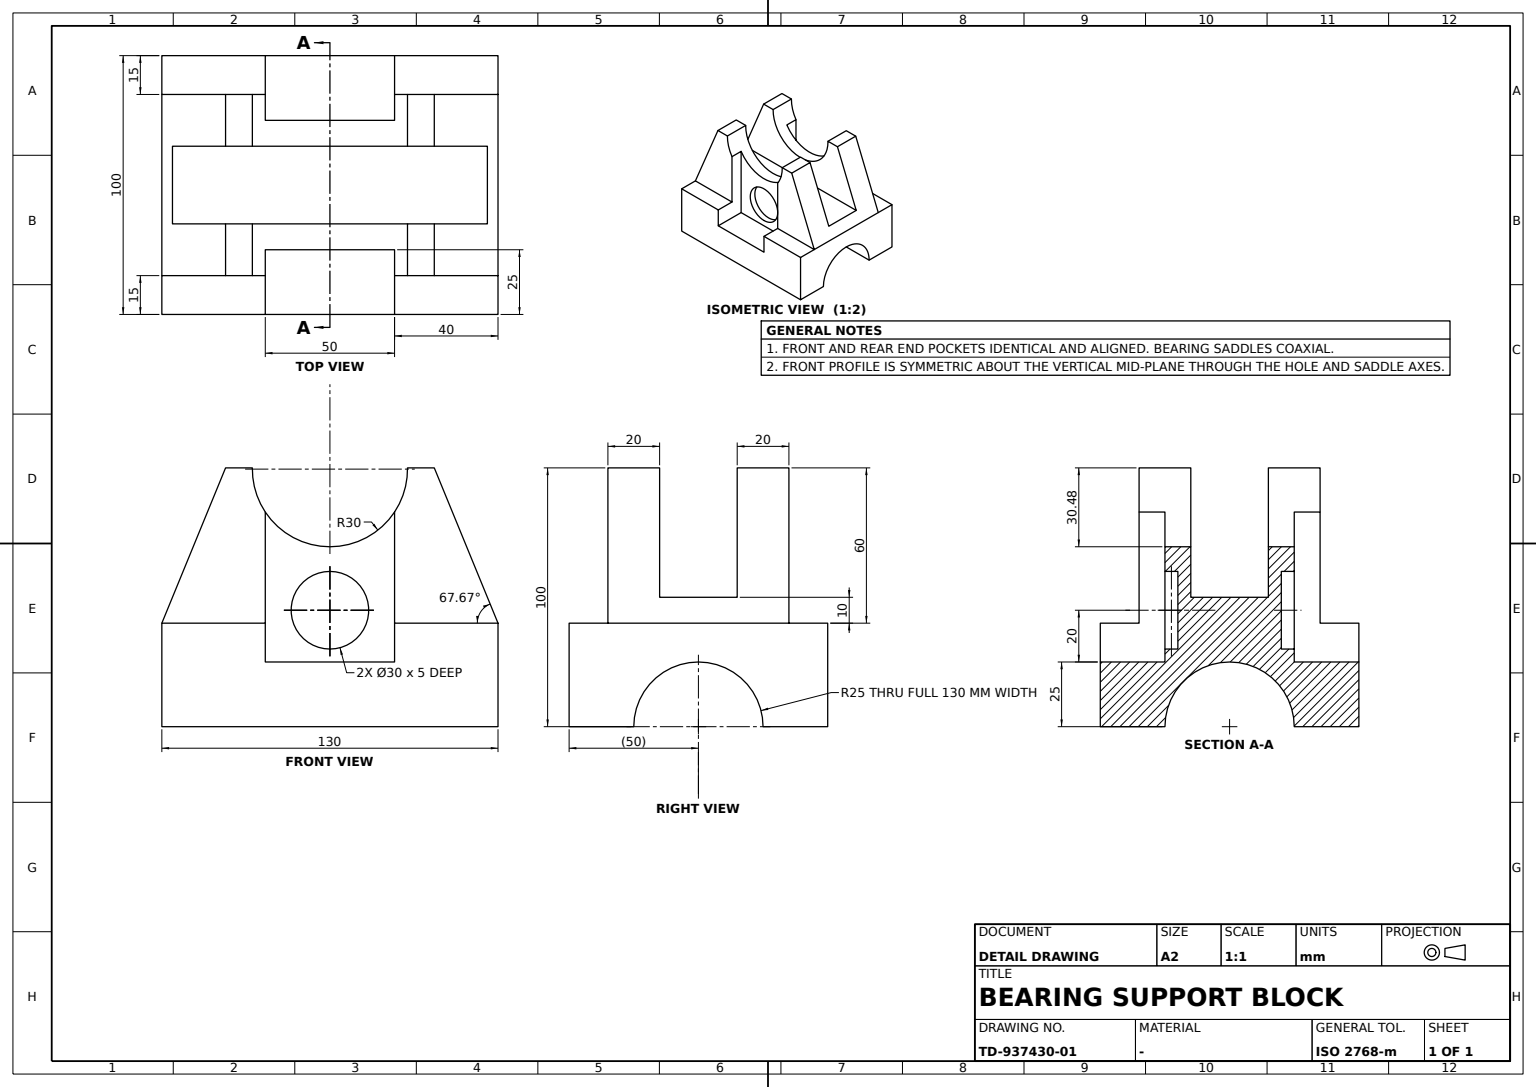
ISO-10303-21;
HEADER;
FILE_DESCRIPTION((''),'2;1');
FILE_NAME('','',(''),(''),'','','');
FILE_SCHEMA(('AUTOMOTIVE_DESIGN'));
ENDSEC;
DATA;
#1=APPLICATION_CONTEXT('');
#2=PRODUCT_CONTEXT('',#1,'mechanical');
#3=PRODUCT('','','',(#2));
#4=PRODUCT_DEFINITION_FORMATION('','',#3);
#5=PRODUCT_DEFINITION_CONTEXT('',#1,'design');
#6=PRODUCT_DEFINITION('','',#4,#5);
#7=PRODUCT_DEFINITION_SHAPE('','',#6);
#8=(LENGTH_UNIT()NAMED_UNIT(*)SI_UNIT(.MILLI.,.METRE.));
#9=(NAMED_UNIT(*)PLANE_ANGLE_UNIT()SI_UNIT($,.RADIAN.));
#10=(NAMED_UNIT(*)SI_UNIT($,.STERADIAN.)SOLID_ANGLE_UNIT());
#11=UNCERTAINTY_MEASURE_WITH_UNIT(LENGTH_MEASURE(0.005),#8,'distance_accuracy_value','');
#12=(GEOMETRIC_REPRESENTATION_CONTEXT(3)GLOBAL_UNCERTAINTY_ASSIGNED_CONTEXT((#11))GLOBAL_UNIT_ASSIGNED_CONTEXT((#8,#9,#10))REPRESENTATION_CONTEXT('',''));
#13=CARTESIAN_POINT('',(-15.,29.996182,100.));
#14=VERTEX_POINT('',#13);
#15=CARTESIAN_POINT('',(-15.,-29.996182,100.));
#16=VERTEX_POINT('',#15);
#17=CARTESIAN_POINT('',(-15.,0.,99.521385));
#18=DIRECTION('',(-1.,0.,0.));
#19=DIRECTION('',(0.,0.,1.));
#20=AXIS2_PLACEMENT_3D('',#17,#18,#19);
#21=CIRCLE('',#20,30.);
#22=EDGE_CURVE('',#14,#16,#21,.T.);
#23=ORIENTED_EDGE('',*,*,#22,.F.);
#24=CARTESIAN_POINT('',(-35.,29.996182,100.));
#25=VERTEX_POINT('',#24);
#26=DIRECTION('',(1.,0.,0.));
#27=VECTOR('',#26,1000.);
#28=LINE('',#13,#27);
#29=EDGE_CURVE('',#14,#25,#28,.F.);
#30=ORIENTED_EDGE('',*,*,#29,.T.);
#31=CARTESIAN_POINT('',(-35.,25.,82.938261));
#32=VERTEX_POINT('',#31);
#33=CARTESIAN_POINT('',(-35.,0.,99.521385));
#34=DIRECTION('',(0.,0.,-1.));
#35=AXIS2_PLACEMENT_3D('',#33,#26,#34);
#36=CIRCLE('',#35,30.);
#37=EDGE_CURVE('',#32,#25,#36,.T.);
#38=ORIENTED_EDGE('',*,*,#37,.F.);
#39=CARTESIAN_POINT('',(-25.,25.,82.938261));
#40=VERTEX_POINT('',#39);
#41=LINE('',#31,#27);
#42=EDGE_CURVE('',#32,#40,#41,.T.);
#43=ORIENTED_EDGE('',*,*,#42,.T.);
#44=CARTESIAN_POINT('',(-25.,-25.,82.938261));
#45=VERTEX_POINT('',#44);
#46=CARTESIAN_POINT('',(-25.,0.,99.521385));
#47=AXIS2_PLACEMENT_3D('',#46,#26,#34);
#48=CIRCLE('',#47,30.);
#49=EDGE_CURVE('',#45,#40,#48,.T.);
#50=ORIENTED_EDGE('',*,*,#49,.F.);
#51=CARTESIAN_POINT('',(-35.,-25.,82.938261));
#52=VERTEX_POINT('',#51);
#53=LINE('',#51,#27);
#54=EDGE_CURVE('',#52,#45,#53,.T.);
#55=ORIENTED_EDGE('',*,*,#54,.F.);
#56=CARTESIAN_POINT('',(-35.,-29.996182,100.));
#57=VERTEX_POINT('',#56);
#58=EDGE_CURVE('',#57,#52,#36,.T.);
#59=ORIENTED_EDGE('',*,*,#58,.F.);
#60=LINE('',#15,#27);
#61=EDGE_CURVE('',#57,#16,#60,.T.);
#62=ORIENTED_EDGE('',*,*,#61,.T.);
#63=EDGE_LOOP('',(#23,#30,#38,#43,#50,#55,#59,#62));
#64=FACE_BOUND('',#63,.T.);
#65=CARTESIAN_POINT('',(-8.16,0.,99.521385));
#66=DIRECTION('',(0.,1.,0.));
#67=AXIS2_PLACEMENT_3D('',#65,#26,#66);
#68=CYLINDRICAL_SURFACE('',#67,30.);
#69=ADVANCED_FACE('',(#64),#68,.F.);
#70=CARTESIAN_POINT('',(-25.,-25.,25.));
#71=VERTEX_POINT('',#70);
#72=CARTESIAN_POINT('',(-25.,-25.,100.));
#73=VECTOR('',#34,1000.);
#74=LINE('',#72,#73);
#75=EDGE_CURVE('',#45,#71,#74,.T.);
#76=ORIENTED_EDGE('',*,*,#75,.F.);
#77=ORIENTED_EDGE('',*,*,#49,.T.);
#78=CARTESIAN_POINT('',(-25.,25.,25.));
#79=VERTEX_POINT('',#78);
#80=CARTESIAN_POINT('',(-25.,25.,40.));
#81=LINE('',#80,#73);
#82=EDGE_CURVE('',#40,#79,#81,.T.);
#83=ORIENTED_EDGE('',*,*,#82,.T.);
#84=DIRECTION('',(0.,-1.,0.));
#85=VECTOR('',#84,1000.);
#86=LINE('',#78,#85);
#87=EDGE_CURVE('',#79,#71,#86,.T.);
#88=ORIENTED_EDGE('',*,*,#87,.T.);
#89=EDGE_LOOP('',(#76,#77,#83,#88));
#90=FACE_BOUND('',#89,.T.);
#91=CARTESIAN_POINT('',(-25.,0.,30.));
#92=VERTEX_POINT('',#91);
#93=CARTESIAN_POINT('',(-25.,0.,45.));
#94=AXIS2_PLACEMENT_3D('',#93,#26,#34);
#95=CIRCLE('',#94,15.);
#96=EDGE_CURVE('',#92,#92,#95,.T.);
#97=ORIENTED_EDGE('',*,*,#96,.T.);
#98=EDGE_LOOP('',(#97));
#99=FACE_BOUND('',#98,.T.);
#100=CARTESIAN_POINT('',(-25.,25.,100.));
#101=AXIS2_PLACEMENT_3D('',#100,#26,#84);
#102=PLANE('',#101);
#103=ADVANCED_FACE('',(#90,#99),#102,.F.);
#104=CARTESIAN_POINT('',(25.,-65.,0.));
#105=VERTEX_POINT('',#104);
#106=CARTESIAN_POINT('',(25.,65.,0.));
#107=VERTEX_POINT('',#106);
#108=VECTOR('',#66,1000.);
#109=LINE('',#104,#108);
#110=EDGE_CURVE('',#105,#107,#109,.T.);
#111=ORIENTED_EDGE('',*,*,#110,.F.);
#112=CARTESIAN_POINT('',(-25.,-65.,0.));
#113=VERTEX_POINT('',#112);
#114=CARTESIAN_POINT('',(0.,-65.,0.));
#115=AXIS2_PLACEMENT_3D('',#114,#66,#19);
#116=CIRCLE('',#115,25.);
#117=EDGE_CURVE('',#113,#105,#116,.T.);
#118=ORIENTED_EDGE('',*,*,#117,.F.);
#119=CARTESIAN_POINT('',(-25.,65.,0.));
#120=VERTEX_POINT('',#119);
#121=LINE('',#112,#108);
#122=EDGE_CURVE('',#120,#113,#121,.F.);
#123=ORIENTED_EDGE('',*,*,#122,.F.);
#124=CARTESIAN_POINT('',(0.,65.,0.));
#125=AXIS2_PLACEMENT_3D('',#124,#84,#34);
#126=CIRCLE('',#125,25.);
#127=EDGE_CURVE('',#120,#107,#126,.F.);
#128=ORIENTED_EDGE('',*,*,#127,.T.);
#129=EDGE_LOOP('',(#111,#118,#123,#128));
#130=FACE_BOUND('',#129,.T.);
#131=CARTESIAN_POINT('',(0.,-0.66,0.));
#132=AXIS2_PLACEMENT_3D('',#131,#66,#18);
#133=CYLINDRICAL_SURFACE('',#132,25.);
#134=ADVANCED_FACE('',(#130),#133,.F.);
#135=CARTESIAN_POINT('',(50.,-65.,40.));
#136=VERTEX_POINT('',#135);
#137=CARTESIAN_POINT('',(35.,-65.,40.));
#138=VERTEX_POINT('',#137);
#139=CARTESIAN_POINT('',(0.,-65.,40.));
#140=VECTOR('',#18,1000.);
#141=LINE('',#139,#140);
#142=EDGE_CURVE('',#136,#138,#141,.T.);
#143=ORIENTED_EDGE('',*,*,#142,.F.);
#144=CARTESIAN_POINT('',(50.,-25.,40.));
#145=VERTEX_POINT('',#144);
#146=CARTESIAN_POINT('',(50.,0.,40.));
#147=LINE('',#146,#85);
#148=EDGE_CURVE('',#145,#136,#147,.T.);
#149=ORIENTED_EDGE('',*,*,#148,.F.);
#150=CARTESIAN_POINT('',(35.,-25.,40.));
#151=VERTEX_POINT('',#150);
#152=LINE('',#144,#140);
#153=EDGE_CURVE('',#145,#151,#152,.T.);
#154=ORIENTED_EDGE('',*,*,#153,.T.);
#155=CARTESIAN_POINT('',(35.,0.,40.));
#156=LINE('',#155,#85);
#157=EDGE_CURVE('',#151,#138,#156,.T.);
#158=ORIENTED_EDGE('',*,*,#157,.T.);
#159=EDGE_LOOP('',(#143,#149,#154,#158));
#160=FACE_BOUND('',#159,.T.);
#161=CARTESIAN_POINT('',(0.,0.,40.));
#162=AXIS2_PLACEMENT_3D('',#161,#19,#66);
#163=PLANE('',#162);
#164=ADVANCED_FACE('',(#160),#163,.T.);
#165=CARTESIAN_POINT('',(15.,-29.996182,100.));
#166=VERTEX_POINT('',#165);
#167=CARTESIAN_POINT('',(35.,-29.996182,100.));
#168=VERTEX_POINT('',#167);
#169=LINE('',#167,#27);
#170=EDGE_CURVE('',#166,#168,#169,.T.);
#171=ORIENTED_EDGE('',*,*,#170,.T.);
#172=CARTESIAN_POINT('',(35.,-25.,82.938261));
#173=VERTEX_POINT('',#172);
#174=CARTESIAN_POINT('',(35.,0.,99.521385));
#175=AXIS2_PLACEMENT_3D('',#174,#18,#19);
#176=CIRCLE('',#175,30.);
#177=EDGE_CURVE('',#168,#173,#176,.F.);
#178=ORIENTED_EDGE('',*,*,#177,.T.);
#179=CARTESIAN_POINT('',(25.,-25.,82.938261));
#180=VERTEX_POINT('',#179);
#181=LINE('',#172,#27);
#182=EDGE_CURVE('',#173,#180,#181,.F.);
#183=ORIENTED_EDGE('',*,*,#182,.T.);
#184=CARTESIAN_POINT('',(25.,25.,82.938261));
#185=VERTEX_POINT('',#184);
#186=CARTESIAN_POINT('',(25.,0.,99.521385));
#187=AXIS2_PLACEMENT_3D('',#186,#26,#34);
#188=CIRCLE('',#187,30.);
#189=EDGE_CURVE('',#180,#185,#188,.T.);
#190=ORIENTED_EDGE('',*,*,#189,.T.);
#191=CARTESIAN_POINT('',(35.,25.,82.938261));
#192=VERTEX_POINT('',#191);
#193=LINE('',#191,#27);
#194=EDGE_CURVE('',#192,#185,#193,.F.);
#195=ORIENTED_EDGE('',*,*,#194,.F.);
#196=CARTESIAN_POINT('',(35.,29.996182,100.));
#197=VERTEX_POINT('',#196);
#198=EDGE_CURVE('',#192,#197,#176,.F.);
#199=ORIENTED_EDGE('',*,*,#198,.T.);
#200=CARTESIAN_POINT('',(15.,29.996182,100.));
#201=VERTEX_POINT('',#200);
#202=LINE('',#196,#27);
#203=EDGE_CURVE('',#197,#201,#202,.F.);
#204=ORIENTED_EDGE('',*,*,#203,.T.);
#205=CARTESIAN_POINT('',(15.,0.,99.521385));
#206=AXIS2_PLACEMENT_3D('',#205,#26,#34);
#207=CIRCLE('',#206,30.);
#208=EDGE_CURVE('',#166,#201,#207,.T.);
#209=ORIENTED_EDGE('',*,*,#208,.F.);
#210=EDGE_LOOP('',(#171,#178,#183,#190,#195,#199,#204,#209));
#211=FACE_BOUND('',#210,.T.);
#212=ADVANCED_FACE('',(#211),#68,.F.);
#213=CARTESIAN_POINT('',(-15.,40.357887,100.));
#214=VERTEX_POINT('',#213);
#215=CARTESIAN_POINT('',(-35.,40.357887,100.));
#216=VERTEX_POINT('',#215);
#217=CARTESIAN_POINT('',(35.,40.357887,100.));
#218=LINE('',#217,#140);
#219=EDGE_CURVE('',#214,#216,#218,.T.);
#220=ORIENTED_EDGE('',*,*,#219,.T.);
#221=CARTESIAN_POINT('',(-35.,0.,100.));
#222=LINE('',#221,#108);
#223=EDGE_CURVE('',#25,#216,#222,.T.);
#224=ORIENTED_EDGE('',*,*,#223,.F.);
#225=ORIENTED_EDGE('',*,*,#29,.F.);
#226=CARTESIAN_POINT('',(-15.,0.,100.));
#227=LINE('',#226,#85);
#228=EDGE_CURVE('',#214,#14,#227,.T.);
#229=ORIENTED_EDGE('',*,*,#228,.F.);
#230=EDGE_LOOP('',(#220,#224,#225,#229));
#231=FACE_BOUND('',#230,.T.);
#232=CARTESIAN_POINT('',(0.,0.,100.));
#233=AXIS2_PLACEMENT_3D('',#232,#19,#66);
#234=PLANE('',#233);
#235=ADVANCED_FACE('',(#231),#234,.T.);
#236=CARTESIAN_POINT('',(50.,-25.,25.));
#237=VERTEX_POINT('',#236);
#238=CARTESIAN_POINT('',(25.,-25.,25.));
#239=VERTEX_POINT('',#238);
#240=LINE('',#236,#140);
#241=EDGE_CURVE('',#237,#239,#240,.T.);
#242=ORIENTED_EDGE('',*,*,#241,.T.);
#243=CARTESIAN_POINT('',(25.,-25.,0.));
#244=LINE('',#243,#73);
#245=EDGE_CURVE('',#180,#239,#244,.T.);
#246=ORIENTED_EDGE('',*,*,#245,.F.);
#247=ORIENTED_EDGE('',*,*,#182,.F.);
#248=CARTESIAN_POINT('',(35.,-25.,25.));
#249=LINE('',#248,#73);
#250=EDGE_CURVE('',#173,#151,#249,.T.);
#251=ORIENTED_EDGE('',*,*,#250,.T.);
#252=ORIENTED_EDGE('',*,*,#153,.F.);
#253=CARTESIAN_POINT('',(50.,-25.,0.));
#254=VECTOR('',#19,1000.);
#255=LINE('',#253,#254);
#256=EDGE_CURVE('',#237,#145,#255,.T.);
#257=ORIENTED_EDGE('',*,*,#256,.F.);
#258=EDGE_LOOP('',(#242,#246,#247,#251,#252,#257));
#259=FACE_BOUND('',#258,.T.);
#260=AXIS2_PLACEMENT_3D('',#236,#84,#19);
#261=PLANE('',#260);
#262=ADVANCED_FACE('',(#259),#261,.F.);
#263=CARTESIAN_POINT('',(-15.,-60.892981,50.));
#264=VERTEX_POINT('',#263);
#265=CARTESIAN_POINT('',(15.,-60.892981,50.));
#266=VERTEX_POINT('',#265);
#267=CARTESIAN_POINT('',(35.,-60.892981,50.));
#268=LINE('',#267,#27);
#269=EDGE_CURVE('',#264,#266,#268,.T.);
#270=ORIENTED_EDGE('',*,*,#269,.F.);
#271=CARTESIAN_POINT('',(-15.,-40.357887,100.));
#272=VERTEX_POINT('',#271);
#273=CARTESIAN_POINT('',(-15.,-65.,40.));
#274=DIRECTION('',(0.,-0.379909034,-0.925023852));
#275=VECTOR('',#274,1000.);
#276=LINE('',#273,#275);
#277=EDGE_CURVE('',#272,#264,#276,.T.);
#278=ORIENTED_EDGE('',*,*,#277,.F.);
#279=CARTESIAN_POINT('',(-35.,-40.357887,100.));
#280=VERTEX_POINT('',#279);
#281=CARTESIAN_POINT('',(35.,-40.357887,100.));
#282=LINE('',#281,#140);
#283=EDGE_CURVE('',#272,#280,#282,.T.);
#284=ORIENTED_EDGE('',*,*,#283,.T.);
#285=CARTESIAN_POINT('',(-35.,-65.,40.));
#286=VERTEX_POINT('',#285);
#287=DIRECTION('',(0.,0.379909034,0.925023852));
#288=VECTOR('',#287,1000.);
#289=LINE('',#285,#288);
#290=EDGE_CURVE('',#286,#280,#289,.T.);
#291=ORIENTED_EDGE('',*,*,#290,.F.);
#292=LINE('',#137,#140);
#293=EDGE_CURVE('',#138,#286,#292,.T.);
#294=ORIENTED_EDGE('',*,*,#293,.F.);
#295=VERTEX_POINT('',#281);
#296=CARTESIAN_POINT('',(35.,-46.236986,85.685239));
#297=LINE('',#296,#288);
#298=EDGE_CURVE('',#138,#295,#297,.T.);
#299=ORIENTED_EDGE('',*,*,#298,.T.);
#300=CARTESIAN_POINT('',(15.,-40.357887,100.));
#301=VERTEX_POINT('',#300);
#302=EDGE_CURVE('',#295,#301,#282,.T.);
#303=ORIENTED_EDGE('',*,*,#302,.T.);
#304=CARTESIAN_POINT('',(15.,-42.722737,94.241931));
#305=LINE('',#304,#275);
#306=EDGE_CURVE('',#301,#266,#305,.T.);
#307=ORIENTED_EDGE('',*,*,#306,.T.);
#308=EDGE_LOOP('',(#270,#278,#284,#291,#294,#299,#303,#307));
#309=FACE_BOUND('',#308,.T.);
#310=DIRECTION('',(0.,-0.925023852,0.379909034));
#311=AXIS2_PLACEMENT_3D('',#137,#310,#287);
#312=PLANE('',#311);
#313=ADVANCED_FACE('',(#309),#312,.T.);
#314=CARTESIAN_POINT('',(50.,65.,0.));
#315=VERTEX_POINT('',#314);
#316=CARTESIAN_POINT('',(50.,-65.,0.));
#317=VERTEX_POINT('',#316);
#318=CARTESIAN_POINT('',(50.,0.,0.));
#319=LINE('',#318,#85);
#320=EDGE_CURVE('',#315,#317,#319,.T.);
#321=ORIENTED_EDGE('',*,*,#320,.T.);
#322=LINE('',#114,#140);
#323=EDGE_CURVE('',#317,#105,#322,.T.);
#324=ORIENTED_EDGE('',*,*,#323,.T.);
#325=ORIENTED_EDGE('',*,*,#110,.T.);
#326=LINE('',#124,#27);
#327=EDGE_CURVE('',#107,#315,#326,.T.);
#328=ORIENTED_EDGE('',*,*,#327,.T.);
#329=EDGE_LOOP('',(#321,#324,#325,#328));
#330=FACE_BOUND('',#329,.T.);
#331=CARTESIAN_POINT('',(0.,0.,0.));
#332=AXIS2_PLACEMENT_3D('',#331,#19,#66);
#333=PLANE('',#332);
#334=ADVANCED_FACE('',(#330),#333,.F.);
#335=CARTESIAN_POINT('',(-50.,-65.,0.));
#336=VERTEX_POINT('',#335);
#337=EDGE_CURVE('',#113,#336,#322,.T.);
#338=ORIENTED_EDGE('',*,*,#337,.T.);
#339=CARTESIAN_POINT('',(-50.,65.,0.));
#340=VERTEX_POINT('',#339);
#341=CARTESIAN_POINT('',(-50.,0.,0.));
#342=LINE('',#341,#108);
#343=EDGE_CURVE('',#336,#340,#342,.T.);
#344=ORIENTED_EDGE('',*,*,#343,.T.);
#345=EDGE_CURVE('',#340,#120,#326,.T.);
#346=ORIENTED_EDGE('',*,*,#345,.T.);
#347=ORIENTED_EDGE('',*,*,#122,.T.);
#348=EDGE_LOOP('',(#338,#344,#346,#347));
#349=FACE_BOUND('',#348,.T.);
#350=ADVANCED_FACE('',(#349),#333,.F.);
#351=ORIENTED_EDGE('',*,*,#96,.F.);
#352=EDGE_LOOP('',(#351));
#353=FACE_BOUND('',#352,.T.);
#354=CARTESIAN_POINT('',(-20.,0.,30.));
#355=VERTEX_POINT('',#354);
#356=CARTESIAN_POINT('',(-20.,0.,45.));
#357=AXIS2_PLACEMENT_3D('',#356,#26,#34);
#358=CIRCLE('',#357,15.);
#359=EDGE_CURVE('',#355,#355,#358,.T.);
#360=ORIENTED_EDGE('',*,*,#359,.T.);
#361=EDGE_LOOP('',(#360));
#362=FACE_BOUND('',#361,.T.);
#363=CARTESIAN_POINT('',(24.9,0.,45.));
#364=AXIS2_PLACEMENT_3D('',#363,#18,#66);
#365=CYLINDRICAL_SURFACE('',#364,15.);
#366=ADVANCED_FACE('',(#353,#362),#365,.F.);
#367=ORIENTED_EDGE('',*,*,#203,.F.);
#368=VERTEX_POINT('',#217);
#369=CARTESIAN_POINT('',(35.,0.,100.));
#370=LINE('',#369,#85);
#371=EDGE_CURVE('',#368,#197,#370,.T.);
#372=ORIENTED_EDGE('',*,*,#371,.F.);
#373=CARTESIAN_POINT('',(15.,40.357887,100.));
#374=VERTEX_POINT('',#373);
#375=EDGE_CURVE('',#368,#374,#218,.T.);
#376=ORIENTED_EDGE('',*,*,#375,.T.);
#377=CARTESIAN_POINT('',(15.,65.,100.));
#378=LINE('',#377,#85);
#379=EDGE_CURVE('',#374,#201,#378,.T.);
#380=ORIENTED_EDGE('',*,*,#379,.T.);
#381=EDGE_LOOP('',(#367,#372,#376,#380));
#382=FACE_BOUND('',#381,.T.);
#383=ADVANCED_FACE('',(#382),#234,.T.);
#384=CARTESIAN_POINT('',(-50.,-25.,25.));
#385=VERTEX_POINT('',#384);
#386=CARTESIAN_POINT('',(-50.,25.,25.));
#387=VERTEX_POINT('',#386);
#388=CARTESIAN_POINT('',(-50.,-65.,25.));
#389=LINE('',#388,#108);
#390=EDGE_CURVE('',#385,#387,#389,.T.);
#391=ORIENTED_EDGE('',*,*,#390,.F.);
#392=EDGE_CURVE('',#71,#385,#240,.T.);
#393=ORIENTED_EDGE('',*,*,#392,.F.);
#394=ORIENTED_EDGE('',*,*,#87,.F.);
#395=CARTESIAN_POINT('',(50.,25.,25.));
#396=LINE('',#395,#27);
#397=EDGE_CURVE('',#387,#79,#396,.T.);
#398=ORIENTED_EDGE('',*,*,#397,.F.);
#399=EDGE_LOOP('',(#391,#393,#394,#398));
#400=FACE_BOUND('',#399,.T.);
#401=AXIS2_PLACEMENT_3D('',#395,#34,#84);
#402=PLANE('',#401);
#403=ADVANCED_FACE('',(#400),#402,.F.);
#404=CARTESIAN_POINT('',(50.,25.,40.));
#405=VERTEX_POINT('',#404);
#406=VERTEX_POINT('',#395);
#407=CARTESIAN_POINT('',(50.,25.,0.));
#408=LINE('',#407,#73);
#409=EDGE_CURVE('',#405,#406,#408,.T.);
#410=ORIENTED_EDGE('',*,*,#409,.T.);
#411=CARTESIAN_POINT('',(50.,65.,25.));
#412=LINE('',#411,#85);
#413=EDGE_CURVE('',#406,#237,#412,.T.);
#414=ORIENTED_EDGE('',*,*,#413,.T.);
#415=ORIENTED_EDGE('',*,*,#256,.T.);
#416=ORIENTED_EDGE('',*,*,#148,.T.);
#417=LINE('',#316,#254);
#418=EDGE_CURVE('',#317,#136,#417,.T.);
#419=ORIENTED_EDGE('',*,*,#418,.F.);
#420=ORIENTED_EDGE('',*,*,#320,.F.);
#421=CARTESIAN_POINT('',(50.,65.,40.));
#422=VERTEX_POINT('',#421);
#423=LINE('',#314,#254);
#424=EDGE_CURVE('',#315,#422,#423,.T.);
#425=ORIENTED_EDGE('',*,*,#424,.T.);
#426=EDGE_CURVE('',#422,#405,#147,.T.);
#427=ORIENTED_EDGE('',*,*,#426,.T.);
#428=EDGE_LOOP('',(#410,#414,#415,#416,#419,#420,#425,#427));
#429=FACE_BOUND('',#428,.T.);
#430=AXIS2_PLACEMENT_3D('',#314,#18,#84);
#431=PLANE('',#430);
#432=ADVANCED_FACE('',(#429),#431,.F.);
#433=ORIENTED_EDGE('',*,*,#189,.F.);
#434=ORIENTED_EDGE('',*,*,#245,.T.);
#435=CARTESIAN_POINT('',(25.,25.,25.));
#436=VERTEX_POINT('',#435);
#437=LINE('',#435,#85);
#438=EDGE_CURVE('',#436,#239,#437,.T.);
#439=ORIENTED_EDGE('',*,*,#438,.F.);
#440=CARTESIAN_POINT('',(25.,25.,40.));
#441=LINE('',#440,#73);
#442=EDGE_CURVE('',#185,#436,#441,.T.);
#443=ORIENTED_EDGE('',*,*,#442,.F.);
#444=EDGE_LOOP('',(#433,#434,#439,#443));
#445=FACE_BOUND('',#444,.T.);
#446=CARTESIAN_POINT('',(25.,0.,30.));
#447=VERTEX_POINT('',#446);
#448=CARTESIAN_POINT('',(25.,0.,45.));
#449=AXIS2_PLACEMENT_3D('',#448,#26,#34);
#450=CIRCLE('',#449,15.);
#451=EDGE_CURVE('',#447,#447,#450,.T.);
#452=ORIENTED_EDGE('',*,*,#451,.F.);
#453=EDGE_LOOP('',(#452));
#454=FACE_BOUND('',#453,.T.);
#455=CARTESIAN_POINT('',(25.,0.,0.));
#456=AXIS2_PLACEMENT_3D('',#455,#26,#66);
#457=PLANE('',#456);
#458=ADVANCED_FACE('',(#445,#454),#457,.T.);
#459=CARTESIAN_POINT('',(35.,25.,40.));
#460=VERTEX_POINT('',#459);
#461=CARTESIAN_POINT('',(0.,25.,40.));
#462=LINE('',#461,#140);
#463=EDGE_CURVE('',#405,#460,#462,.T.);
#464=ORIENTED_EDGE('',*,*,#463,.F.);
#465=ORIENTED_EDGE('',*,*,#426,.F.);
#466=CARTESIAN_POINT('',(35.,65.,40.));
#467=VERTEX_POINT('',#466);
#468=CARTESIAN_POINT('',(0.,65.,40.));
#469=LINE('',#468,#27);
#470=EDGE_CURVE('',#467,#422,#469,.T.);
#471=ORIENTED_EDGE('',*,*,#470,.F.);
#472=EDGE_CURVE('',#467,#460,#156,.T.);
#473=ORIENTED_EDGE('',*,*,#472,.T.);
#474=EDGE_LOOP('',(#464,#465,#471,#473));
#475=FACE_BOUND('',#474,.T.);
#476=ADVANCED_FACE('',(#475),#163,.T.);
#477=CARTESIAN_POINT('',(15.,60.892981,50.));
#478=VERTEX_POINT('',#477);
#479=CARTESIAN_POINT('',(15.,65.,50.));
#480=LINE('',#479,#85);
#481=EDGE_CURVE('',#478,#266,#480,.T.);
#482=ORIENTED_EDGE('',*,*,#481,.F.);
#483=CARTESIAN_POINT('',(-15.,60.892981,50.));
#484=VERTEX_POINT('',#483);
#485=CARTESIAN_POINT('',(35.,60.892981,50.));
#486=LINE('',#485,#27);
#487=EDGE_CURVE('',#484,#478,#486,.T.);
#488=ORIENTED_EDGE('',*,*,#487,.F.);
#489=CARTESIAN_POINT('',(-15.,65.,50.));
#490=LINE('',#489,#85);
#491=EDGE_CURVE('',#484,#264,#490,.T.);
#492=ORIENTED_EDGE('',*,*,#491,.T.);
#493=ORIENTED_EDGE('',*,*,#269,.T.);
#494=EDGE_LOOP('',(#482,#488,#492,#493));
#495=FACE_BOUND('',#494,.T.);
#496=AXIS2_PLACEMENT_3D('',#489,#34,#26);
#497=PLANE('',#496);
#498=ADVANCED_FACE('',(#495),#497,.F.);
#499=EDGE_CURVE('',#168,#295,#370,.T.);
#500=ORIENTED_EDGE('',*,*,#499,.T.);
#501=ORIENTED_EDGE('',*,*,#298,.F.);
#502=ORIENTED_EDGE('',*,*,#157,.F.);
#503=ORIENTED_EDGE('',*,*,#250,.F.);
#504=ORIENTED_EDGE('',*,*,#177,.F.);
#505=EDGE_LOOP('',(#500,#501,#502,#503,#504));
#506=FACE_BOUND('',#505,.T.);
#507=AXIS2_PLACEMENT_3D('',#466,#18,#84);
#508=PLANE('',#507);
#509=ADVANCED_FACE('',(#506),#508,.F.);
#510=ORIENTED_EDGE('',*,*,#327,.F.);
#511=ORIENTED_EDGE('',*,*,#127,.F.);
#512=ORIENTED_EDGE('',*,*,#345,.F.);
#513=CARTESIAN_POINT('',(-50.,65.,40.));
#514=VERTEX_POINT('',#513);
#515=LINE('',#339,#254);
#516=EDGE_CURVE('',#340,#514,#515,.T.);
#517=ORIENTED_EDGE('',*,*,#516,.T.);
#518=CARTESIAN_POINT('',(-35.,65.,40.));
#519=VERTEX_POINT('',#518);
#520=EDGE_CURVE('',#514,#519,#469,.T.);
#521=ORIENTED_EDGE('',*,*,#520,.T.);
#522=LINE('',#466,#140);
#523=EDGE_CURVE('',#467,#519,#522,.T.);
#524=ORIENTED_EDGE('',*,*,#523,.F.);
#525=ORIENTED_EDGE('',*,*,#470,.T.);
#526=ORIENTED_EDGE('',*,*,#424,.F.);
#527=EDGE_LOOP('',(#510,#511,#512,#517,#521,#524,#525,#526));
#528=FACE_BOUND('',#527,.T.);
#529=AXIS2_PLACEMENT_3D('',#339,#84,#26);
#530=PLANE('',#529);
#531=ADVANCED_FACE('',(#528),#530,.F.);
#532=LINE('',#395,#140);
#533=EDGE_CURVE('',#406,#436,#532,.T.);
#534=ORIENTED_EDGE('',*,*,#533,.F.);
#535=ORIENTED_EDGE('',*,*,#409,.F.);
#536=ORIENTED_EDGE('',*,*,#463,.T.);
#537=LINE('',#459,#73);
#538=EDGE_CURVE('',#192,#460,#537,.T.);
#539=ORIENTED_EDGE('',*,*,#538,.F.);
#540=ORIENTED_EDGE('',*,*,#194,.T.);
#541=ORIENTED_EDGE('',*,*,#442,.T.);
#542=EDGE_LOOP('',(#534,#535,#536,#539,#540,#541));
#543=FACE_BOUND('',#542,.T.);
#544=AXIS2_PLACEMENT_3D('',#404,#66,#34);
#545=PLANE('',#544);
#546=ADVANCED_FACE('',(#543),#545,.F.);
#547=ORIENTED_EDGE('',*,*,#397,.T.);
#548=ORIENTED_EDGE('',*,*,#82,.F.);
#549=ORIENTED_EDGE('',*,*,#42,.F.);
#550=CARTESIAN_POINT('',(-35.,25.,40.));
#551=VERTEX_POINT('',#550);
#552=LINE('',#550,#73);
#553=EDGE_CURVE('',#32,#551,#552,.T.);
#554=ORIENTED_EDGE('',*,*,#553,.T.);
#555=CARTESIAN_POINT('',(-50.,25.,40.));
#556=VERTEX_POINT('',#555);
#557=LINE('',#404,#27);
#558=EDGE_CURVE('',#556,#551,#557,.T.);
#559=ORIENTED_EDGE('',*,*,#558,.F.);
#560=LINE('',#555,#73);
#561=EDGE_CURVE('',#556,#387,#560,.T.);
#562=ORIENTED_EDGE('',*,*,#561,.T.);
#563=EDGE_LOOP('',(#547,#548,#549,#554,#559,#562));
#564=FACE_BOUND('',#563,.T.);
#565=ADVANCED_FACE('',(#564),#545,.F.);
#566=CARTESIAN_POINT('',(20.,0.,60.));
#567=VERTEX_POINT('',#566);
#568=CARTESIAN_POINT('',(20.,0.,45.));
#569=AXIS2_PLACEMENT_3D('',#568,#18,#19);
#570=CIRCLE('',#569,15.);
#571=EDGE_CURVE('',#567,#567,#570,.T.);
#572=ORIENTED_EDGE('',*,*,#571,.F.);
#573=EDGE_LOOP('',(#572));
#574=FACE_BOUND('',#573,.T.);
#575=AXIS2_PLACEMENT_3D('',#568,#18,#66);
#576=PLANE('',#575);
#577=ADVANCED_FACE('',(#574),#576,.F.);
#578=ORIENTED_EDGE('',*,*,#359,.F.);
#579=EDGE_LOOP('',(#578));
#580=FACE_BOUND('',#579,.T.);
#581=AXIS2_PLACEMENT_3D('',#356,#26,#66);
#582=PLANE('',#581);
#583=ADVANCED_FACE('',(#580),#582,.F.);
#584=ORIENTED_EDGE('',*,*,#241,.F.);
#585=ORIENTED_EDGE('',*,*,#413,.F.);
#586=ORIENTED_EDGE('',*,*,#533,.T.);
#587=ORIENTED_EDGE('',*,*,#438,.T.);
#588=EDGE_LOOP('',(#584,#585,#586,#587));
#589=FACE_BOUND('',#588,.T.);
#590=ADVANCED_FACE('',(#589),#402,.F.);
#591=ORIENTED_EDGE('',*,*,#117,.T.);
#592=ORIENTED_EDGE('',*,*,#323,.F.);
#593=ORIENTED_EDGE('',*,*,#418,.T.);
#594=ORIENTED_EDGE('',*,*,#142,.T.);
#595=ORIENTED_EDGE('',*,*,#293,.T.);
#596=CARTESIAN_POINT('',(-50.,-65.,40.));
#597=VERTEX_POINT('',#596);
#598=EDGE_CURVE('',#286,#597,#141,.T.);
#599=ORIENTED_EDGE('',*,*,#598,.T.);
#600=LINE('',#335,#254);
#601=EDGE_CURVE('',#336,#597,#600,.T.);
#602=ORIENTED_EDGE('',*,*,#601,.F.);
#603=ORIENTED_EDGE('',*,*,#337,.F.);
#604=EDGE_LOOP('',(#591,#592,#593,#594,#595,#599,#602,#603));
#605=FACE_BOUND('',#604,.T.);
#606=AXIS2_PLACEMENT_3D('',#316,#66,#18);
#607=PLANE('',#606);
#608=ADVANCED_FACE('',(#605),#607,.F.);
#609=ORIENTED_EDGE('',*,*,#558,.T.);
#610=CARTESIAN_POINT('',(-35.,0.,40.));
#611=LINE('',#610,#108);
#612=EDGE_CURVE('',#551,#519,#611,.T.);
#613=ORIENTED_EDGE('',*,*,#612,.T.);
#614=ORIENTED_EDGE('',*,*,#520,.F.);
#615=CARTESIAN_POINT('',(-50.,0.,40.));
#616=LINE('',#615,#108);
#617=EDGE_CURVE('',#556,#514,#616,.T.);
#618=ORIENTED_EDGE('',*,*,#617,.F.);
#619=EDGE_LOOP('',(#609,#613,#614,#618));
#620=FACE_BOUND('',#619,.T.);
#621=ADVANCED_FACE('',(#620),#163,.T.);
#622=ORIENTED_EDGE('',*,*,#553,.F.);
#623=ORIENTED_EDGE('',*,*,#37,.T.);
#624=ORIENTED_EDGE('',*,*,#223,.T.);
#625=DIRECTION('',(0.,-0.379909034,0.925023852));
#626=VECTOR('',#625,1000.);
#627=LINE('',#518,#626);
#628=EDGE_CURVE('',#519,#216,#627,.T.);
#629=ORIENTED_EDGE('',*,*,#628,.F.);
#630=ORIENTED_EDGE('',*,*,#612,.F.);
#631=EDGE_LOOP('',(#622,#623,#624,#629,#630));
#632=FACE_BOUND('',#631,.T.);
#633=AXIS2_PLACEMENT_3D('',#285,#26,#66);
#634=PLANE('',#633);
#635=ADVANCED_FACE('',(#632),#634,.F.);
#636=ORIENTED_EDGE('',*,*,#601,.T.);
#637=CARTESIAN_POINT('',(-50.,-25.,40.));
#638=VERTEX_POINT('',#637);
#639=EDGE_CURVE('',#597,#638,#616,.T.);
#640=ORIENTED_EDGE('',*,*,#639,.T.);
#641=CARTESIAN_POINT('',(-50.,-25.,0.));
#642=LINE('',#641,#73);
#643=EDGE_CURVE('',#638,#385,#642,.T.);
#644=ORIENTED_EDGE('',*,*,#643,.T.);
#645=ORIENTED_EDGE('',*,*,#390,.T.);
#646=ORIENTED_EDGE('',*,*,#561,.F.);
#647=ORIENTED_EDGE('',*,*,#617,.T.);
#648=ORIENTED_EDGE('',*,*,#516,.F.);
#649=ORIENTED_EDGE('',*,*,#343,.F.);
#650=EDGE_LOOP('',(#636,#640,#644,#645,#646,#647,#648,#649));
#651=FACE_BOUND('',#650,.T.);
#652=AXIS2_PLACEMENT_3D('',#335,#26,#66);
#653=PLANE('',#652);
#654=ADVANCED_FACE('',(#651),#653,.F.);
#655=ORIENTED_EDGE('',*,*,#628,.T.);
#656=ORIENTED_EDGE('',*,*,#219,.F.);
#657=CARTESIAN_POINT('',(-15.,65.,40.));
#658=DIRECTION('',(0.,0.379909034,-0.925023852));
#659=VECTOR('',#658,1000.);
#660=LINE('',#657,#659);
#661=EDGE_CURVE('',#214,#484,#660,.T.);
#662=ORIENTED_EDGE('',*,*,#661,.T.);
#663=ORIENTED_EDGE('',*,*,#487,.T.);
#664=CARTESIAN_POINT('',(15.,61.485751,48.556691));
#665=LINE('',#664,#659);
#666=EDGE_CURVE('',#374,#478,#665,.T.);
#667=ORIENTED_EDGE('',*,*,#666,.F.);
#668=ORIENTED_EDGE('',*,*,#375,.F.);
#669=LINE('',#466,#626);
#670=EDGE_CURVE('',#467,#368,#669,.T.);
#671=ORIENTED_EDGE('',*,*,#670,.F.);
#672=ORIENTED_EDGE('',*,*,#523,.T.);
#673=EDGE_LOOP('',(#655,#656,#662,#663,#667,#668,#671,#672));
#674=FACE_BOUND('',#673,.T.);
#675=DIRECTION('',(0.,-0.925023852,-0.379909034));
#676=AXIS2_PLACEMENT_3D('',#466,#675,#625);
#677=PLANE('',#676);
#678=ADVANCED_FACE('',(#674),#677,.F.);
#679=ORIENTED_EDGE('',*,*,#170,.F.);
#680=EDGE_CURVE('',#166,#301,#378,.T.);
#681=ORIENTED_EDGE('',*,*,#680,.T.);
#682=ORIENTED_EDGE('',*,*,#302,.F.);
#683=ORIENTED_EDGE('',*,*,#499,.F.);
#684=EDGE_LOOP('',(#679,#681,#682,#683));
#685=FACE_BOUND('',#684,.T.);
#686=ADVANCED_FACE('',(#685),#234,.T.);
#687=CARTESIAN_POINT('',(-35.,-25.,40.));
#688=VERTEX_POINT('',#687);
#689=EDGE_CURVE('',#286,#688,#611,.T.);
#690=ORIENTED_EDGE('',*,*,#689,.T.);
#691=EDGE_CURVE('',#688,#638,#152,.T.);
#692=ORIENTED_EDGE('',*,*,#691,.T.);
#693=ORIENTED_EDGE('',*,*,#639,.F.);
#694=ORIENTED_EDGE('',*,*,#598,.F.);
#695=EDGE_LOOP('',(#690,#692,#693,#694));
#696=FACE_BOUND('',#695,.T.);
#697=ADVANCED_FACE('',(#696),#163,.T.);
#698=EDGE_CURVE('',#280,#57,#222,.T.);
#699=ORIENTED_EDGE('',*,*,#698,.T.);
#700=ORIENTED_EDGE('',*,*,#58,.T.);
#701=LINE('',#687,#73);
#702=EDGE_CURVE('',#52,#688,#701,.T.);
#703=ORIENTED_EDGE('',*,*,#702,.T.);
#704=ORIENTED_EDGE('',*,*,#689,.F.);
#705=ORIENTED_EDGE('',*,*,#290,.T.);
#706=EDGE_LOOP('',(#699,#700,#703,#704,#705));
#707=FACE_BOUND('',#706,.T.);
#708=ADVANCED_FACE('',(#707),#634,.F.);
#709=ORIENTED_EDGE('',*,*,#451,.T.);
#710=EDGE_LOOP('',(#709));
#711=FACE_BOUND('',#710,.T.);
#712=ORIENTED_EDGE('',*,*,#571,.T.);
#713=EDGE_LOOP('',(#712));
#714=FACE_BOUND('',#713,.T.);
#715=ADVANCED_FACE('',(#711,#714),#365,.F.);
#716=ORIENTED_EDGE('',*,*,#228,.T.);
#717=ORIENTED_EDGE('',*,*,#22,.T.);
#718=EDGE_CURVE('',#16,#272,#227,.T.);
#719=ORIENTED_EDGE('',*,*,#718,.T.);
#720=ORIENTED_EDGE('',*,*,#277,.T.);
#721=ORIENTED_EDGE('',*,*,#491,.F.);
#722=ORIENTED_EDGE('',*,*,#661,.F.);
#723=EDGE_LOOP('',(#716,#717,#719,#720,#721,#722));
#724=FACE_BOUND('',#723,.T.);
#725=CARTESIAN_POINT('',(-15.,65.,100.));
#726=AXIS2_PLACEMENT_3D('',#725,#18,#34);
#727=PLANE('',#726);
#728=ADVANCED_FACE('',(#724),#727,.F.);
#729=ORIENTED_EDGE('',*,*,#702,.F.);
#730=ORIENTED_EDGE('',*,*,#54,.T.);
#731=ORIENTED_EDGE('',*,*,#75,.T.);
#732=ORIENTED_EDGE('',*,*,#392,.T.);
#733=ORIENTED_EDGE('',*,*,#643,.F.);
#734=ORIENTED_EDGE('',*,*,#691,.F.);
#735=EDGE_LOOP('',(#729,#730,#731,#732,#733,#734));
#736=FACE_BOUND('',#735,.T.);
#737=ADVANCED_FACE('',(#736),#261,.F.);
#738=ORIENTED_EDGE('',*,*,#670,.T.);
#739=ORIENTED_EDGE('',*,*,#371,.T.);
#740=ORIENTED_EDGE('',*,*,#198,.F.);
#741=ORIENTED_EDGE('',*,*,#538,.T.);
#742=ORIENTED_EDGE('',*,*,#472,.F.);
#743=EDGE_LOOP('',(#738,#739,#740,#741,#742));
#744=FACE_BOUND('',#743,.T.);
#745=ADVANCED_FACE('',(#744),#508,.F.);
#746=ORIENTED_EDGE('',*,*,#306,.F.);
#747=ORIENTED_EDGE('',*,*,#680,.F.);
#748=ORIENTED_EDGE('',*,*,#208,.T.);
#749=ORIENTED_EDGE('',*,*,#379,.F.);
#750=ORIENTED_EDGE('',*,*,#666,.T.);
#751=ORIENTED_EDGE('',*,*,#481,.T.);
#752=EDGE_LOOP('',(#746,#747,#748,#749,#750,#751));
#753=FACE_BOUND('',#752,.T.);
#754=AXIS2_PLACEMENT_3D('',#479,#26,#19);
#755=PLANE('',#754);
#756=ADVANCED_FACE('',(#753),#755,.F.);
#757=ORIENTED_EDGE('',*,*,#283,.F.);
#758=ORIENTED_EDGE('',*,*,#718,.F.);
#759=ORIENTED_EDGE('',*,*,#61,.F.);
#760=ORIENTED_EDGE('',*,*,#698,.F.);
#761=EDGE_LOOP('',(#757,#758,#759,#760));
#762=FACE_BOUND('',#761,.T.);
#763=ADVANCED_FACE('',(#762),#234,.T.);
#764=CLOSED_SHELL('',(#69,#103,#134,#164,#212,#235,#262,#313,#334,#350,#366,#383,#403,#432,#458,#476,#498,#509,#531,#546,#565,#577,#583,#590,#608,#621,#635,#654,#678,#686,#697,#708,#715,#728,#737,#745,#756,#763));
#765=MANIFOLD_SOLID_BREP('',#764);
#766=ADVANCED_BREP_SHAPE_REPRESENTATION('',(#765),#12);
#767=SHAPE_DEFINITION_REPRESENTATION(#7,#766);
ENDSEC;
END-ISO-10303-21;
